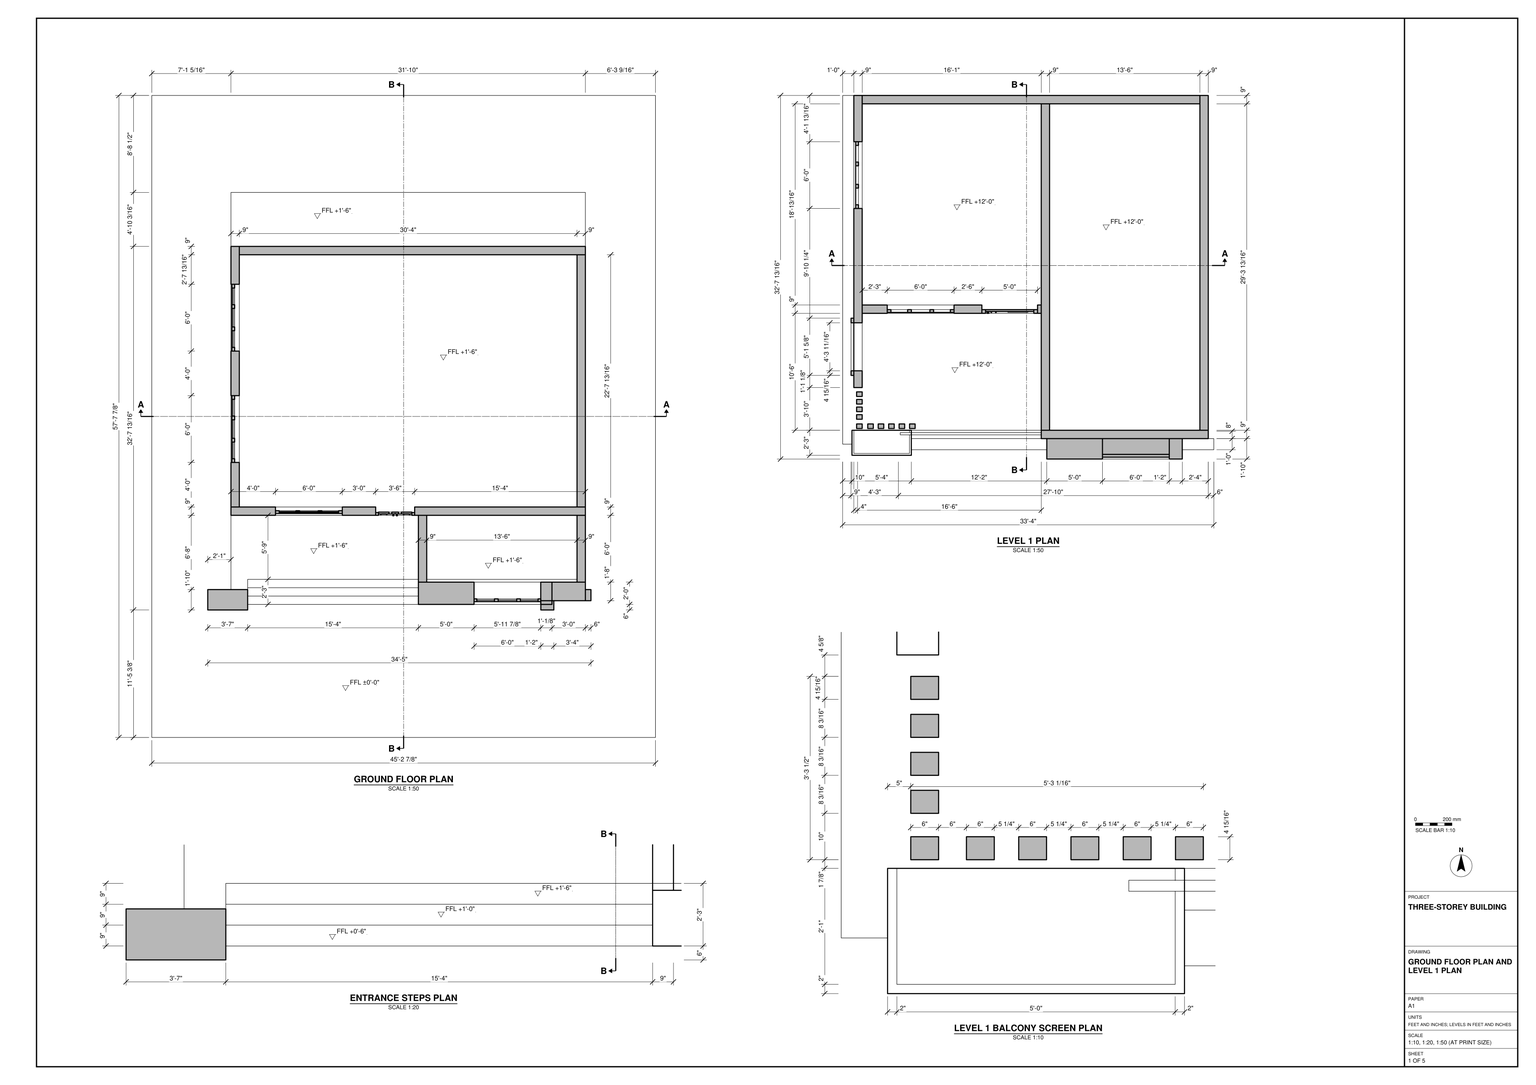
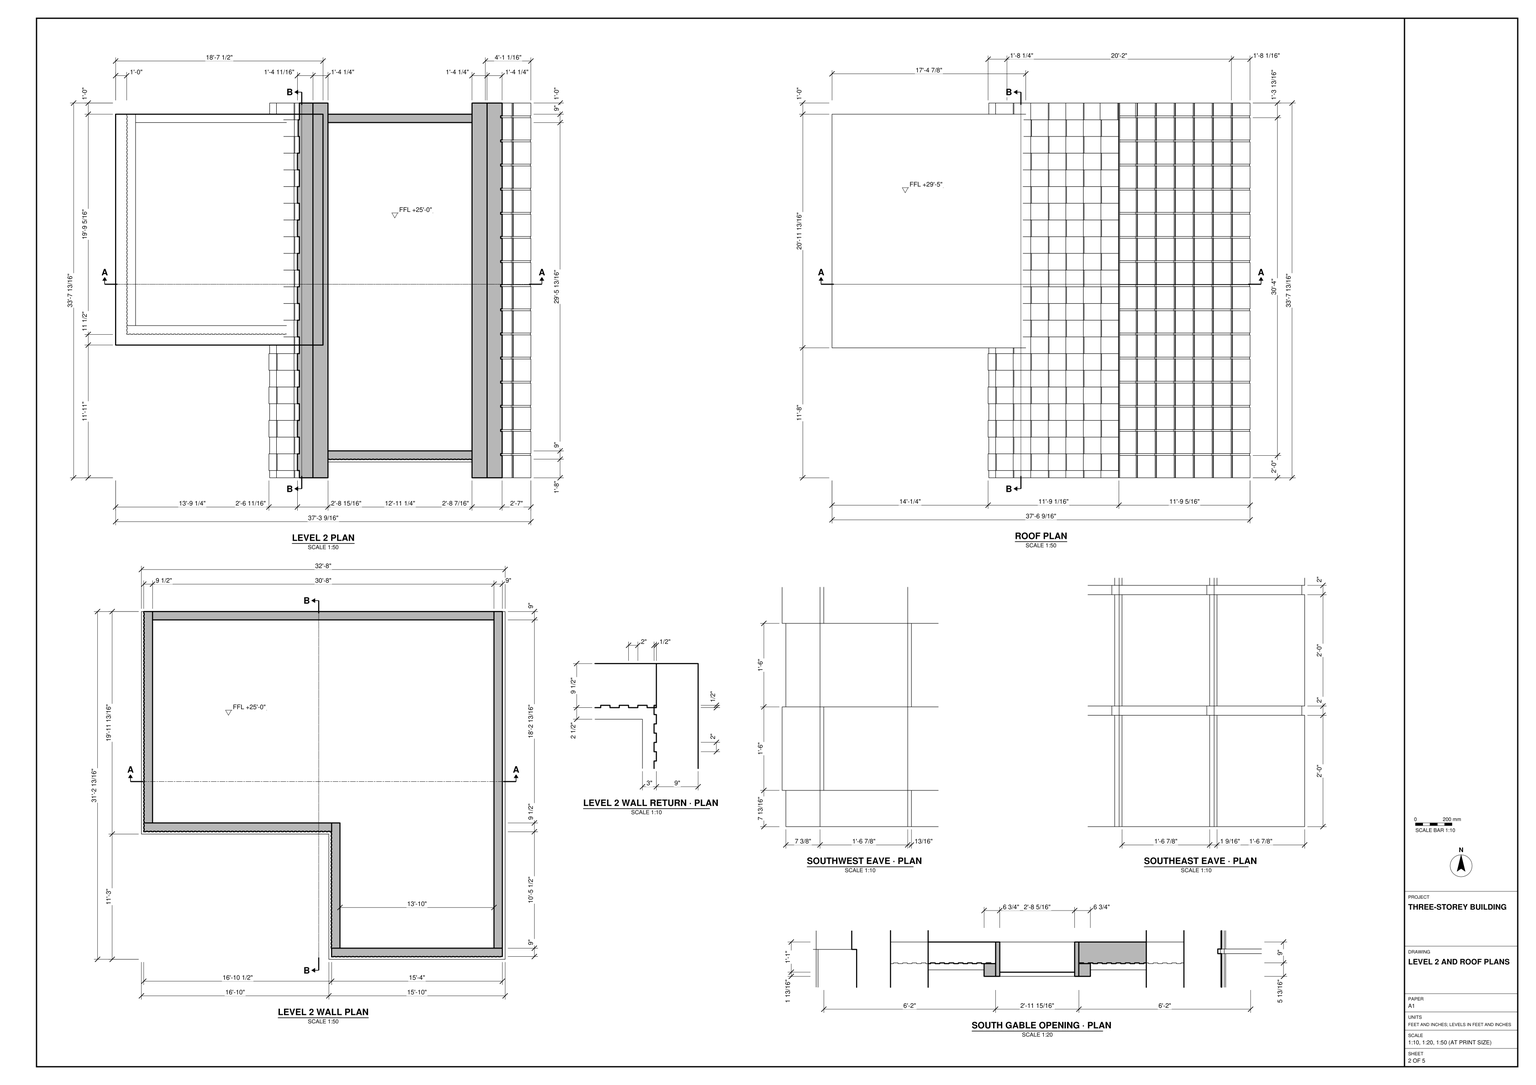
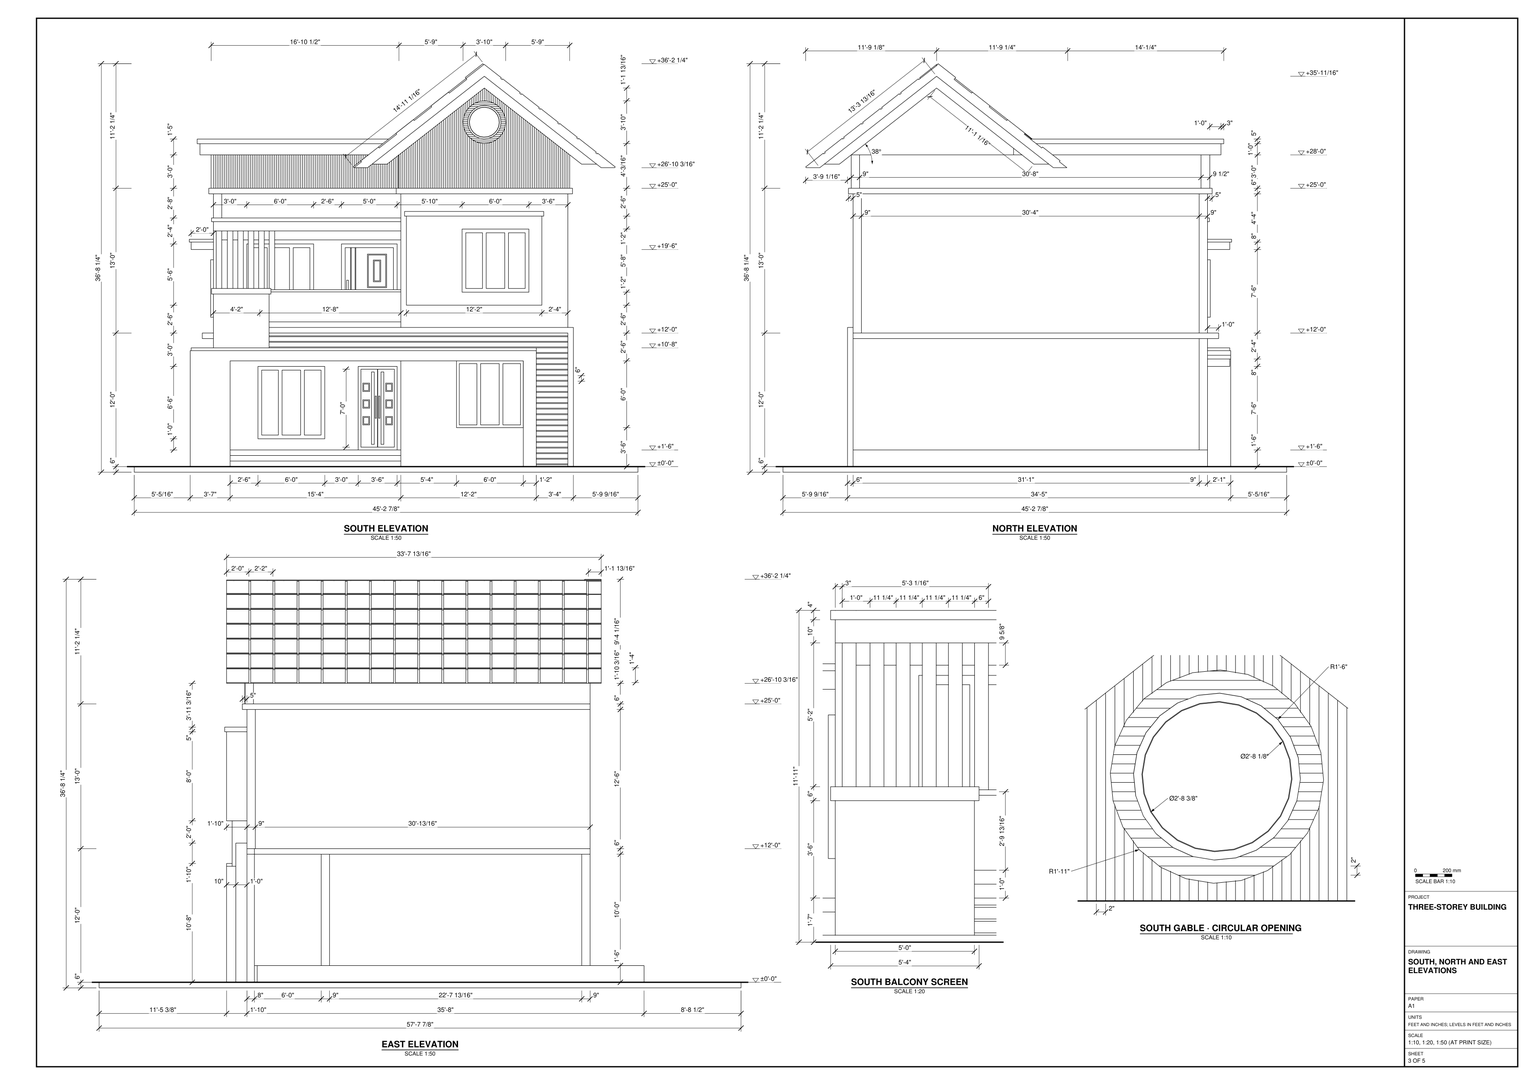
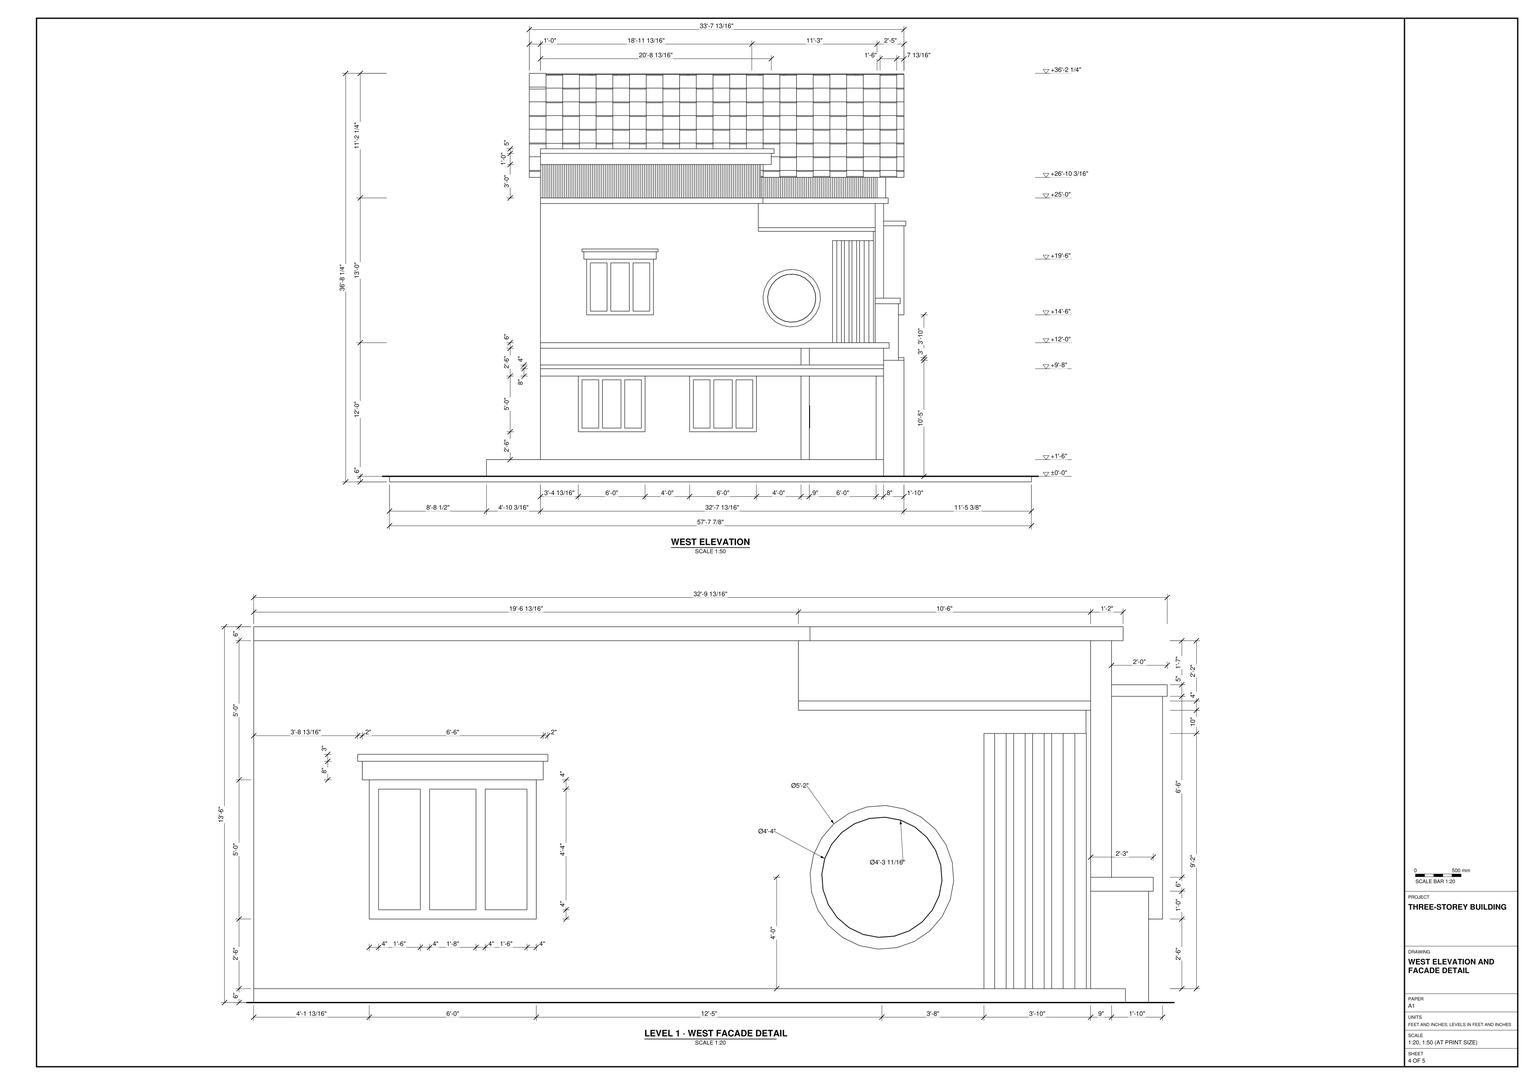
Build the three-storey building and its rectangular site base in SketchUp using task_files/diagram_01.pdf. Work in feet and inches. Including the base, the model is 45'-2 7/8" wide, 57'-7 7/8" deep and 36'-8 1/4" high. Use ±0'-0" as the ground datum, with Level 1 at +12'-0" and Level 2 at +25'-0". The entrance steps rise from the ground datum to the raised ground floor at +1'-6".

Set out the floor slabs and walls from the plans, keeping the 9" wall thicknesses where marked. On the south side, recess the entrance beside the projecting room and place the doors and windows in their drawn wall planes. At Level 1, model the front balcony with its solid corner base and returning vertical screen. Distinguish the recessed balcony openings from the window in the projecting frame to their right.

Follow the L-shaped Level 2 wall plan. Model the flat roof to the west and the adjoining pitched roof with its ridge running north–south. Include the eave projections, roof divisions and framed circular opening beneath the south gable peak. Keep walls, slabs, roof and any furniture or joinery pieces in separate groups or components, and use components for repeated parts. Any decor or loose items shown may be suitable library components. Save one SketchUp model as output_files/gabled_three_storey_building_with_screened_balcony.skp.

# SketchUp Ruby script. Lengths in inches.
U = 1.inch
M = Sketchup.active_model
def pt(a) = Geom::Point3d.new(a.map { |v| v * U })
def face(e, loops, mat)
  f = e.add_face(loops[0].map { |a| pt(a) })
  loops[1..].each { |l| e.add_face(l.map { |a| pt(a) }).erase! }
  f.material = f.back_material = mat if mat
  f
end
# faces: each face lists its corners as indices into pts; further lists are holes
def faces(e, pts, list, mat = nil) = list.each { |f| face(e, (f[0].is_a?(Array) ? f : [f]).map { |l| l.map { |i| pts[i] } }, mat) }
# xy, xz, yz: faces in a plane at the given z, y or x. An outline is a flat list of corners, or four numbers for a rectangle; further outlines are holes
def ring(l) = l.size == 4 ? [[l[0], l[1]], [l[2], l[1]], [l[2], l[3]], [l[0], l[3]]] : l.each_slice(2).to_a
def flat(e, list, mat, &to3) = list.each { |f| face(e, (f[0].is_a?(Array) ? f : [f]).map { |l| ring(l).map { |u, v| to3.(u, v) } }, mat) }
def xy(e, z, list, mat = nil) = flat(e, list, mat) { |x, y| [x, y, z] }
def xz(e, y, list, mat = nil) = flat(e, list, mat) { |x, z| [x, y, z] }
def yz(e, x, list, mat = nil) = flat(e, list, mat) { |y, z| [x, y, z] }
def lines(e, pts, list) = list.each { |a, b| e.add_line(pt(pts[a]), pt(pts[b])) }
# prism: a flat outline (further loops are holes) pulled along v
def prism(e, loops, v, mat = nil)
  f = face(e, loops, mat); d = Geom::Vector3d.new(v.map { |x| x * U })
  f.pushpull(f.normal.samedirection?(d) ? d.length : -d.length)
end
def box(e, o, s, mat = nil) = prism(e, [[o, [o[0] + s[0], o[1], o[2]], [o[0] + s[0], o[1] + s[1], o[2]], [o[0], o[1] + s[1], o[2]]]], [0, 0, s[2]], mat)
def at(x, y, z, deg = 0) = Geom::Transformation.translation(pt([x, y, z])) * Geom::Transformation.rotation(ORIGIN, Z_AXIS, deg.degrees)
def axes(o, x, y, z) = Geom::Transformation.new([*x, 0, *y, 0, *z, 0, *pt(o).to_a, 1])
def part(name) = M.definitions.add(name)
# library, detail: a bought-in or finely detailed component or shape, given as its bounding box
def library(name, o, s) = part(name).tap { |d| box(d.entities, o, s) }
def detail(e, o, s) = box(e.add_group.entities, o, s)
def put(e, d, t, mat = nil) = e.add_instance(d, t).tap { |i| i.material = mat if mat }
def group(e, t, mat = nil) = e.add_group.tap { |g| g.transformation = t; g.material = mat if mat }.entities
root = M.entities
M.materials.add("[Color M00]").color = [255, 255, 255]
M.materials.add("[Color M01]").color = [226, 226, 226]
M.materials.add("[Color M02]").color = [198, 198, 198]
M.materials.add("[Color M03]").color = [170, 170, 170]
M.materials.add("[Color M04]").color = [142, 142, 142]
M.materials.add("[Color M05]").color = [114, 114, 114]
M.materials.add("[Color M06]").color = [86, 86, 86]
M.materials.add("[Metal Silver]").color = [234, 233, 238]
M.materials.add("[Translucent Glass Gray]").color = [128, 128, 128]
M.materials.add("[Wood Cherry Original]").color = [152, 86, 42]
c1 = library("Group\#7",[-5,0,0],[69,0.75,0.75])
c2 = library("Group\#92",[-5,0,0],[69,0.75,0.75])
c3 = library("Group\#93",[-5,0,0],[69,0.75,0.75])
c4 = library("Group\#94",[-5,0,0],[69,0.75,0.75])
c5 = library("Group\#95",[-5,0,0],[69,0.75,0.75])
c6 = library("Group\#96",[-5,0,0],[69,0.75,0.75])
c7 = library("Group\#97",[-5,0,0],[69,0.75,0.75])
c8 = library("Group\#98",[-5,0,0],[69,0.75,0.75])
c9 = library("Group\#99",[-5,0,0],[69,0.75,0.75])
c10 = library("Group\#100",[-5,0,0],[69,0.75,0.75])
c11 = library("Group\#101",[-5,0,0],[69,0.75,0.75])
c12 = library("Group\#13",[0,-0.5,0],[36,2.5,84])
c13 = part("Group\#16")
prism(c13.entities,[[[0,2,23.9375],[0,2,22.2],[0,0.74,22.2],[0,0.74,1.74],[0,2,1.74],[0,2,0],[0,0,0],[0,0,23.9375]]],[1.1875,0,0])
c14 = library("Group\#18",[0,0,0],[64,1.125,1.125])
c15 = library("Group\#25",[0,0,0],[1.125,64,1.125])
c16 = library("Group\#30",[0,0,0],[1,64,1])
c17 = library("Group\#56",[0,0,0],[158,2.375,2.375])
c18 = library("Group\#66",[0,-1,0],[52,3,88])
c19 = part("Group\#73")
box(c19.entities,[0,0,0],[6,4.96,110])
c20 = library("Group\#80",[0,-5.8,-36],[184,14.8,108])
c21 = library("Group\#78",[0,-0.5,0],[45.98,5.5,45.98])
c22 = library("Group\#83",[-0.5,0,0],[9.5,135,36])
c23 = library("Group\#90",[-0.8,0,0],[282.36,403.8125,112.04])
g1 = group(root,at(0,0,0))
box(g1,[0,0,0],[542.875,691.875,6])
g2 = group(root,at(47.33,167.375,6),"[Color M05]")
xy(g2,0,[[38,-8,38,420,420,420,420,3,56,3,56,-8]])
xy(g2,18,[[38,-8,56,-8,56,3,420,3,420,420,38,420]],"[Color M00]")
xz(g2,-8,[[38,0,56,18]])
xz(g2,3,[[56,0,420,18]])
xz(g2,420,[[38,0,420,18]])
yz(g2,38,[[-8,0,420,18]])
yz(g2,56,[[-8,0,3,18]])
yz(g2,420,[[3,0,420,18]])
g3 = group(root,at(47.33,239.375,24),"[Color M01]")
prism(g3,[[[194,9,0],[38,9,0],[38,9,120],[420,9,120],[420,9,0],[236,9,0],[236,9,90],[194,9,90]],[[158,9,90],[86,9,90],[86,9,12],[158,9,12]]],[0,-9,0])
g4 = group(root,at(287.33,143.375,6),"[Color M01]")
xy(g4,0,[[0,0,144,24]])
xy(g4,42,[[60,0,131.9,24]])
xy(g4,114,[[0,0,60,12],[131.9,0,144,12]])
xy(g4,138,[[0,12,60,24],[131.9,12,144,24]])
xz(g4,0,[[0,0,144,0,144,114,131.9,114,131.9,42,60,42,60,114,0,114]])
xz(g4,12,[[0,114,60,138],[131.9,114,144,138]])
xz(g4,24,[[0,0,0,138,60,138,60,42,131.9,42,131.9,138,144,138,144,0]])
yz(g4,0,[[0,0,0,114,12,114,12,138,24,138,24,0]])
yz(g4,60,[[0,42,24,42,24,138,12,138,12,114,0,114]])
yz(g4,131.9,[[0,42,0,114,12,114,12,138,24,138,24,42]])
yz(g4,144,[[0,0,24,0,24,138,12,138,12,114,0,114]])
g5 = group(root,at(287.33,167.375,24))
box(g5,[0,0,0],[9,72,120])
g6 = group(root,at(347.33,146.375,48),"[Wood Cherry Original]")
prism(g6,[[[72,3,0],[0,3,0],[0,3,72],[72,3,72]],[[46,3,3],[46,3,69],[26,3,69],[26,3,3]],[[22,3,3],[22,3,69],[3,3,69],[3,3,3]],[[69,3,69],[50,3,69],[50,3,3],[69,3,3]]],[0,-3,0])
put(root,c1,at(352.33,147.5,114.5))
put(root,c2,at(352.33,147.5,108.5))
put(root,c3,at(352.33,147.5,102.5))
put(root,c4,at(352.33,147.5,96.5))
put(root,c5,at(352.33,147.5,90.5))
put(root,c6,at(352.33,147.5,84.5))
put(root,c7,at(352.33,147.5,78.5))
put(root,c8,at(352.33,147.5,72.5))
put(root,c9,at(352.33,147.5,66.5))
put(root,c10,at(352.33,147.5,60.5))
put(root,c11,at(352.33,147.5,54.5))
g7 = group(root,at(397.33,146.375,51),"[Translucent Glass Gray]")
xz(g7,0,[[0,0,19,66]])
g8 = group(root,at(373.33,146.375,51),"[Translucent Glass Gray]")
xz(g8,0,[[0,0,20,66]])
g9 = group(root,at(350.33,146.375,51),"[Translucent Glass Gray]")
xz(g9,0,[[0,0,19,66]])
g10 = group(root,at(287.33,147.375,6),"[Color M04]")
xy(g10,0,[[144,0,180,20]])
xy(g10,2,[[144,0,180,0.5]])
xy(g10,3,[[144,0,180,0.5]])
xy(g10,8,[[144,0,180,0.5]])
xy(g10,9,[[144,0,180,0.5]])
xy(g10,14,[[144,0,180,0.5]])
xy(g10,15,[[144,0,180,0.5]])
xy(g10,20,[[144,0,180,0.5]])
xy(g10,21,[[144,0,180,0.5]])
xy(g10,26,[[144,0,180,0.5]])
xy(g10,27,[[144,0,180,0.5]])
xy(g10,32,[[144,0,180,0.5]])
xy(g10,33,[[144,0,180,0.5]])
xy(g10,38,[[144,0,180,0.5]])
xy(g10,39,[[144,0,180,0.5]])
xy(g10,44,[[144,0,180,0.5]])
xy(g10,45,[[144,0,180,0.5]])
xy(g10,50,[[144,0,180,0.5]])
xy(g10,51,[[144,0,180,0.5]])
xy(g10,56,[[144,0,180,0.5]])
xy(g10,57,[[144,0,180,0.5]])
xy(g10,62,[[144,0,180,0.5]])
xy(g10,63,[[144,0,180,0.5]])
xy(g10,68,[[144,0,180,0.5]])
xy(g10,69,[[144,0,180,0.5]])
xy(g10,74,[[144,0,180,0.5]])
xy(g10,75,[[144,0,180,0.5]])
xy(g10,80,[[144,0,180,0.5]])
xy(g10,81,[[144,0,180,0.5]])
xy(g10,86,[[144,0,180,0.5]])
xy(g10,87,[[144,0,180,0.5]])
xy(g10,92,[[144,0,180,0.5]])
xy(g10,93,[[144,0,180,0.5]])
xy(g10,98,[[144,0,180,0.5]])
xy(g10,99,[[144,0,180,0.5]])
xy(g10,104,[[144,0,180,0.5]])
xy(g10,105,[[144,0,180,0.5]])
xy(g10,110,[[144,0,180,0.5]])
xy(g10,111,[[144,0,180,0.5]])
xy(g10,114,[[0,0,0,12,60,12,60,20,144,20,144,0]])
xy(g10,116,[[0,0,180,0.5]])
xy(g10,117,[[0,0,180,0.5]])
xy(g10,122,[[0,0,180,0.5]])
xy(g10,123,[[0,0,180,0.5]])
xy(g10,125,[[-154,0,0,12]])
xy(g10,128,[[-154,0,180,0.5]])
xy(g10,129,[[-154,0,180,0.5]])
xy(g10,134,[[-154,0,180,0.5]])
xy(g10,135,[[-154,0,180,0.5]])
xy(g10,140,[[-154,0,180,0.5]])
xy(g10,141,[[-154,0,180,0.5]])
xy(g10,144,[[-154,0,180,0,180,20,60,20,60,12,-154,12]])
xz(g10,0,[[144,0,180,2],[144,3,180,8],[144,9,180,14],[144,15,180,20],[144,21,180,26],
  [144,27,180,32],[144,33,180,38],[144,39,180,44],[144,45,180,50],[144,51,180,56],
  [144,57,180,62],[144,63,180,68],[144,69,180,74],[144,75,180,80],[144,81,180,86],
  [144,87,180,92],[144,93,180,98],[144,99,180,104],[144,105,180,110],[144,111,180,111,180,116,0,116,0,114,144,114],
  [0,117,180,122],[0,123,180,123,180,128,-154,128,-154,125,0,125],[-154,129,180,134],[-154,135,180,140],[-154,141,180,144]])
xz(g10,0.5,[[144,2,180,3],[144,8,180,9],[144,14,180,15],[144,20,180,21],[144,26,180,27],
  [144,32,180,33],[144,38,180,39],[144,44,180,45],[144,50,180,51],[144,56,180,57],
  [144,62,180,63],[144,68,180,69],[144,74,180,75],[144,80,180,81],[144,86,180,87],
  [144,92,180,93],[144,98,180,99],[144,104,180,105],[144,110,180,111],[0,116,180,117],
  [0,122,180,123],[-154,128,180,129],[-154,134,180,135],[-154,140,180,141]])
xz(g10,12,[[0,114,0,125,-154,125,-154,144,60,144,60,114]])
xz(g10,20,[[144,0,144,114,60,114,60,144,180,144,180,0]])
yz(g10,-154,[[0,125,0,128,0.5,128,0.5,129,0,129,0,134,0.5,134,0.5,135,0,135,0,140,0.5,140,0.5,141,0,141,0,144,12,144,12,125]])
yz(g10,0,[[0,114,0,116,0.5,116,0.5,117,0,117,0,122,0.5,122,0.5,123,0,123,0,125,12,125,12,114]])
yz(g10,60,[[12,114,20,144]])
yz(g10,144,[[0,0,0,2,0.5,2,0.5,3,0,3,0,8,0.5,8,0.5,9,0,9,0,14,0.5,14,0.5,15,0,15,0,20,0.5,20,0.5,21,0,21,0,26,0.5,26,0.5,27,0,27,0,32,0.5,32,0.5,33,0,33,0,38,0.5,38,0.5,39,0,39,0,44,0.5,44,0.5,45,0,45,0,50,0.5,50,0.5,51,0,51,0,56,0.5,56,0.5,57,0,57,0,62,0.5,62,0.5,63,0,63,0,68,0.5,68,0.5,69,0,69,0,74,0.5,74,0.5,75,0,75,0,80,0.5,80,0.5,81,0,81,0,86,0.5,86,0.5,87,0,87,0,92,0.5,92,0.5,93,0,93,0,98,0.5,98,0.5,99,0,99,0,104,0.5,104,0.5,105,0,105,0,110,0.5,110,0.5,111,0,111,0,114,20,114,20,0]])
yz(g10,180,[[0,0,20,0,20,144,0,144,0,141,0.5,141,0.5,140,0,140,0,135,0.5,135,0.5,134,0,134,0,129,0.5,129,0.5,128,0,128,0,123,0.5,123,0.5,122,0,122,0,117,0.5,117,0.5,116,0,116,0,111,0.5,111,0.5,110,0,110,0,105,0.5,105,0.5,104,0,104,0,99,0.5,99,0.5,98,0,98,0,93,0.5,93,0.5,92,0,92,0,87,0.5,87,0.5,86,0,86,0,81,0.5,81,0.5,80,0,80,0,75,0.5,75,0.5,74,0,74,0,69,0.5,69,0.5,68,0,68,0,63,0.5,63,0.5,62,0,62,0,57,0.5,57,0.5,56,0,56,0,51,0.5,51,0.5,50,0,50,0,45,0.5,45,0.5,44,0,44,0,39,0.5,39,0.5,38,0,38,0,33,0.5,33,0.5,32,0,32,0,27,0.5,27,0.5,26,0,26,0,21,0.5,21,0.5,20,0,20,0,15,0.5,15,0.5,14,0,14,0,9,0.5,9,0.5,8,0,8,0,3,0.5,3,0.5,2,0,2]])
g11 = group(root,at(241.33,239.375,24),"[Wood Cherry Original]")
prism(g11,[[[42,0,90],[0,0,90],[0,0,0],[42,0,0]],[[3,0,3],[3,0,87],[39,0,87],[39,0,3]]],[0,3,0])
put(root,c12,at(244.33,240.875,27),"[Wood Cherry Original]")
g12 = group(root,at(265.98,240.875,30),"[Translucent Glass Gray]")
xz(g12,0,[[0,0,3,78]])
g13 = group(root,at(255.68,240.875,30),"[Translucent Glass Gray]")
xz(g13,0,[[0,0,3,78]])
put(root,c13,at(259.73,238.875,58.14),"[Metal Silver]")
put(root,c13,at(263.54,238.875,58.14),"[Metal Silver]")
g14 = group(root,at(133.33,241.375,36),"[Wood Cherry Original]")
prism(g14,[[[72,0,78],[0,0,78],[0,0,0],[72,0,0]],[[46,0,4],[26,0,4],[26,0,74],[46,0,74]],[[22,0,74],[22,0,4],[4,0,4],[4,0,74]],[[50,0,4],[50,0,74],[68,0,74],[68,0,4]]],[0,3,0])
put(root,c14,at(137.33,242.3125,107.07))
put(root,c14,at(137.33,242.3125,101.07))
put(root,c14,at(137.33,242.3125,95.07))
put(root,c14,at(137.33,242.3125,89.07))
put(root,c14,at(137.33,242.3125,83.07))
put(root,c14,at(137.33,242.3125,77.07))
put(root,c14,at(137.33,242.3125,71.07))
put(root,c14,at(137.33,242.3125,65.07))
put(root,c14,at(137.33,242.3125,59.07))
put(root,c14,at(137.33,242.3125,53.07))
put(root,c14,at(137.33,242.3125,47.07))
put(root,c14,at(137.33,242.3125,41.07))
put(root,c14,at(137.33,242.3125,35.07))
put(root,c14,at(137.33,242.3125,29.07))
put(root,c14,at(137.33,242.3125,23.07))
put(root,c14,at(137.33,242.3125,17.07))
g15 = group(root,at(183.33,241.375,40),"[Translucent Glass Gray]")
xz(g15,0,[[0,0,18,70]])
g16 = group(root,at(159.33,241.375,40),"[Translucent Glass Gray]")
xz(g16,0,[[0,0,20,70]])
g17 = group(root,at(137.33,241.375,40),"[Translucent Glass Gray]")
xz(g17,0,[[0,0,18,70]])
g18 = group(root,at(85.33,137.375,6),"[Color M05]")
xy(g18,0,[[-25,0,18,22],[334,0,348,10]])
xy(g18,114,[[18,0,18,22,202,22,202,10,334,10,334,0]])
xy(g18,125,[[-25,0,348,0,348,10,202,10,202,22,-25,22]])
xz(g18,0,[[-25,0,18,0,18,114,334,114,334,0,348,0,348,125,-25,125]])
xz(g18,10,[[334,0,334,114,202,114,202,125,348,125,348,0]])
xz(g18,22,[[-25,0,-25,125,202,125,202,114,18,114,18,0]])
yz(g18,-25,[[0,0,22,125]])
yz(g18,18,[[0,0,22,114]])
yz(g18,202,[[10,114,22,125]])
yz(g18,334,[[0,0,10,114]])
yz(g18,348,[[0,0,10,125]])
g19 = group(root,at(85.33,248.375,24),"[Color M01]")
prism(g19,[[[0,280.8125,0],[0,0,0],[0,0,120],[0,280.8125,120]],[[0,48,30],[0,120,30],[0,120,90],[0,48,90]],[[0,240,30],[0,240,90],[0,168,90],[0,168,30]]],[9,0,0])
g20 = group(root,at(86.33,296.375,54),"[Wood Cherry Original]")
prism(g20,[[[0,72,0],[0,0,0],[0,0,60],[0,72,60]],[[0,26,4],[0,46,4],[0,46,56],[0,26,56]],[[0,22,4],[0,22,56],[0,4,56],[0,4,4]],[[0,50,56],[0,50,4],[0,68,4],[0,68,56]]],[3,0,0])
put(root,c15,at(87.27,300.375,104.45))
put(root,c15,at(87.27,300.375,98.45))
put(root,c15,at(87.27,300.375,92.45))
put(root,c15,at(87.27,300.375,86.45))
put(root,c15,at(87.27,300.375,80.45))
put(root,c15,at(87.27,300.375,74.45))
put(root,c15,at(87.27,300.375,68.45))
put(root,c15,at(87.27,300.375,62.45))
put(root,c15,at(87.27,300.375,56.45))
g21 = group(root,at(86.33,300.375,58),"[Translucent Glass Gray]")
yz(g21,0,[[0,0,18,52]])
g22 = group(root,at(86.33,322.375,58),"[Translucent Glass Gray]")
yz(g22,0,[[0,0,20,52]])
g23 = group(root,at(86.33,346.375,58),"[Translucent Glass Gray]")
yz(g23,0,[[0,0,18,52]])
g24 = group(root,at(86.33,416.375,54),"[Wood Cherry Original]")
prism(g24,[[[0,0,60],[0,72,60],[0,72,0],[0,0,0]],[[0,26,56],[0,26,4],[0,46,4],[0,46,56]],[[0,68,56],[0,50,56],[0,50,4],[0,68,4]],[[0,4,4],[0,22,4],[0,22,56],[0,4,56]]],[3,0,0])
put(root,c16,at(87.33,420.375,104.78))
put(root,c16,at(87.33,420.375,98.78))
put(root,c16,at(87.33,420.375,92.78))
put(root,c16,at(87.33,420.375,86.78))
put(root,c16,at(87.33,420.375,80.78))
put(root,c16,at(87.33,420.375,74.78))
put(root,c16,at(87.33,420.375,68.78))
put(root,c16,at(87.33,420.375,62.78))
g25 = group(root,at(86.33,420.375,58),"[Translucent Glass Gray]")
yz(g25,0,[[0,0,18,52]])
g26 = group(root,at(86.33,442.375,58),"[Translucent Glass Gray]")
yz(g26,0,[[0,0,20,52]])
g27 = group(root,at(86.33,466.375,58),"[Translucent Glass Gray]")
yz(g27,0,[[0,0,18,52]])
g28 = group(root,at(94.33,520.1875,24),"[Color M01]")
box(g28,[0,0,0],[373,9,120])
g29 = group(root,at(458.33,248.375,24),"[Color M01]")
box(g29,[0,0,0],[9,271.8125,120])
g30 = group(root,at(61.33,137.375,131),"[Color M05]")
box(g30,[0,0,0],[372,6,3])
g31 = group(root,at(85.33,239.375,144),"[Color M05]")
xy(g31,0,[[-12,-86,-12,289.8125,382,289.8125,382,-80,0,-80,0,-86]])
xy(g31,6,[[-12,-86,0,-86,0,-80,382,-80,382,289.8125,-12,289.8125]],"[Color M00]")
xz(g31,-86,[[-12,0,0,6]])
xz(g31,-80,[[0,0,382,6]])
xz(g31,289.8125,[[-12,0,382,6]])
yz(g31,-12,[[-86,0,289.8125,6]])
yz(g31,0,[[-86,0,-80,6]])
yz(g31,382,[[-80,0,289.8125,6]])
g32 = group(root,at(208.08,147.375,6))
prism(g32,[[[-74.75,0,144],[259.25,0,144],[259.25,0,0],[265.25,0,0],[265.25,0,150],[-74.75,0,150]]],[0,12,0])
g33 = group(root,at(61.33,167.375,126))
box(g33,[24,-8,0],[202,80,18])
g34 = group(root,at(61.33,239.375,114))
box(g34,[0,-80,0],[24,369.8125,8])
g35 = group(root,at(60.33,239.375,122),"[Color M05]")
box(g35,[0,-80,0],[25,369.8125,4])
g36 = group(root,at(85.33,143.375,131),"[Color M02]")
xy(g36,0,[[0,0,60,16]])
xy(g36,19,[[0,16,4,25]])
xy(g36,31,[[4,16,60,25]])
xy(g36,61,[[0,0,60,25]])
xz(g36,0,[[0,0,60,61]])
xz(g36,16,[[0,0,0,19,4,19,4,31,60,31,60,0]])
xz(g36,25,[[0,19,0,61,60,61,60,31,4,31,4,19]])
yz(g36,0,[[0,0,0,61,25,61,25,19,16,19,16,0]])
yz(g36,4,[[16,19,25,31]])
yz(g36,60,[[0,0,16,0,16,31,25,31,25,61,0,61]])
g37 = group(root,at(458.33,167.375,24),"[Color M01]")
box(g37,[0,0,0],[9,72,120])
g38 = group(root,at(287.33,159.375,150),"[Color M01]")
box(g38,[0,0,0],[180,9,150])
g39 = group(root,at(287.33,168.375,150),"[Color M01]")
box(g39,[0,0,0],[9,351.8125,150])
g40 = group(root,at(458.33,168.375,150),"[Color M01]")
box(g40,[0,0,0],[9,360.8125,150])
g41 = group(root,at(76.33,294.375,150),"[Color M01]")
prism(g41,[[[211,9,0],[207,9,0],[207,9,96],[147,9,96],[147,9,0],[18,9,0],[18,9,150],[211,9,150]],[[117,9,96],[45,9,96],[45,9,30],[117,9,30]]],[0,-9,0])
g42 = group(root,at(85.33,255.375,150),"[Color M01]")
xy(g42,0,[[0,-41,9,273.8125]])
xy(g42,30,[[0,152,9,224]])
xy(g42,90,[[0,152,9,224]])
xy(g42,110,[[0,-85,0,-41,9,-41,9,39,202,39,202,-85]])
xy(g42,120,[[0,-85,202,39]])
xy(g42,150,[[0,39,9,273.8125]])
xz(g42,-85,[[0,110,202,120]])
xz(g42,-41,[[0,0,9,110]])
xz(g42,39,[[9,110,202,120],[0,120,9,150]])
xz(g42,152,[[0,30,9,90]])
xz(g42,224,[[0,30,9,90]])
xz(g42,273.8125,[[0,0,9,150]])
yz(g42,-3,[[[4.67,17.04,-3.4,17.67,-11.03,20.36,-17.71,24.93,-22.97,31.08,-26.47,38.38,-27.96,46.33,-27.33,54.4,-24.64,62.03,-20.07,68.71,-13.92,73.97,-6.62,77.47,1.33,78.96,9.4,78.33,17.03,75.64,23.71,71.07,28.97,64.92,32.47,57.62,33.96,49.67,33.33,41.6,30.64,33.97,26.07,27.29,19.92,22.03,12.62,18.53],[4.4,22.04,11.07,23.28,17.19,26.22,22.35,30.63,26.18,36.23,28.44,42.63,28.96,49.4,27.72,56.07,24.78,62.19,20.37,67.35,14.77,71.18,8.37,73.44,1.6,73.96,-5.07,72.72,-11.19,69.78,-16.35,65.37,-20.18,59.77,-22.44,53.37,-22.96,46.6,-21.72,39.93,-18.78,33.81,-14.37,28.65,-8.77,24.82,-2.37,22.56]]],"[Color M04]")
yz(g42,0,[[[-41,0,-41,110,-85,110,-85,120,39,120,39,150,273.8125,150,273.8125,0],[152,30,224,90],[4.67,17.04,12.62,18.53,19.92,22.03,26.07,27.29,30.64,33.97,33.33,41.6,33.96,49.67,32.47,57.62,28.97,64.92,23.71,71.07,17.03,75.64,9.4,78.33,1.33,78.96,-6.62,77.47,-13.92,73.97,-20.07,68.71,-24.64,62.03,-27.33,54.4,-27.96,46.33,-26.47,38.38,-22.97,31.08,-17.71,24.93,-11.03,20.36,-3.4,17.67]],[[4.67,17.04,-3.4,17.67,-11.03,20.36,-17.71,24.93,-22.97,31.08,-26.47,38.38,-27.96,46.33,-27.33,54.4,-24.64,62.03,-20.07,68.71,-13.92,73.97,-6.62,77.47,1.33,78.96,9.4,78.33,17.03,75.64,23.71,71.07,28.97,64.92,32.47,57.62,33.96,49.67,33.33,41.6,30.64,33.97,26.07,27.29,19.92,22.03,12.62,18.53],[4.4,22.04,11.07,23.28,17.19,26.22,22.35,30.63,26.18,36.23,28.44,42.63,28.96,49.4,27.72,56.07,24.78,62.19,20.37,67.35,14.77,71.18,8.37,73.44,1.6,73.96,-5.07,72.72,-11.19,69.78,-16.35,65.37,-20.18,59.77,-22.44,53.37,-22.96,46.6,-21.72,39.93,-18.78,33.81,-14.37,28.65,-8.77,24.82,-2.37,22.56]]])
yz(g42,0,[[4.39,22.18,11.03,23.42,17.12,26.33,22.24,30.73,26.06,36.29,28.3,42.66,28.82,49.39,27.58,56.03,24.67,62.12,20.27,67.24,14.71,71.06,8.34,73.3,1.61,73.82,-5.03,72.58,-11.12,69.67,-16.24,65.27,-20.06,59.71,-22.3,53.34,-22.82,46.61,-21.58,39.97,-18.67,33.88,-14.27,28.76,-8.71,24.94,-2.34,22.7]],"[Translucent Glass Gray]")
yz(g42,9,[[[-41,0,273.8125,0,273.8125,150,39,150,39,110,-41,110],[152,30,224,90],[4.4,22.04,-2.37,22.56,-8.77,24.82,-14.37,28.65,-18.78,33.81,-21.72,39.93,-22.96,46.6,-22.44,53.37,-20.18,59.77,-16.35,65.37,-11.19,69.78,-5.07,72.72,1.6,73.96,8.37,73.44,14.77,71.18,20.37,67.35,24.78,62.19,27.72,56.07,28.96,49.4,28.44,42.63,26.18,36.23,22.35,30.63,17.19,26.22,11.07,23.28]]])
yz(g42,202,[[-85,110,39,120]])
p = [[0,4.67,17.04],[0,-3.4,17.67],[-3,-3.4,17.67],[-3,4.67,17.04],[0,12.62,18.53],[-3,12.62,18.53],
  [0,-11.03,20.36],[-3,-11.03,20.36],[0,19.92,22.03],[-3,19.92,22.03],[0,-17.71,24.93],[-3,-17.71,24.93],
  [0,-2.37,22.56],[0,4.4,22.04],[-3,4.4,22.04],[-3,-2.37,22.56],[9,-2.37,22.56],[9,4.4,22.04],
  [0,11.07,23.28],[-3,11.07,23.28],[9,11.07,23.28],[0,26.07,27.29],[-3,26.07,27.29],[0,-8.77,24.82],
  [-3,-8.77,24.82],[9,-8.77,24.82],[0,17.19,26.22],[-3,17.19,26.22],[9,17.19,26.22],[0,-14.37,28.65],
  [-3,-14.37,28.65],[9,-14.37,28.65],[0,-22.97,31.08],[-3,-22.97,31.08],[0,22.35,30.63],[-3,22.35,30.63],
  [9,22.35,30.63],[0,30.64,33.97],[-3,30.64,33.97],[0,-18.78,33.81],[-3,-18.78,33.81],[9,-18.78,33.81],
  [0,26.18,36.23],[-3,26.18,36.23],[9,26.18,36.23],[0,-26.47,38.38],[-3,-26.47,38.38],[0,-21.72,39.93],
  [-3,-21.72,39.93],[9,-21.72,39.93],[0,33.33,41.6],[-3,33.33,41.6],[0,28.44,42.63],[-3,28.44,42.63],
  [9,28.44,42.63],[0,-27.96,46.33],[-3,-27.96,46.33],[0,-22.96,46.6],[-3,-22.96,46.6],[9,-22.96,46.6],
  [0,33.96,49.67],[-3,33.96,49.67],[0,28.96,49.4],[-3,28.96,49.4],[9,28.96,49.4],[0,-27.33,54.4],
  [-3,-27.33,54.4],[0,-22.44,53.37],[-3,-22.44,53.37],[9,-22.44,53.37],[0,27.72,56.07],[-3,27.72,56.07],
  [9,27.72,56.07],[0,32.47,57.62],[-3,32.47,57.62],[0,-20.18,59.77],[-3,-20.18,59.77],[9,-20.18,59.77],
  [0,-24.64,62.03],[-3,-24.64,62.03],[0,24.78,62.19],[-3,24.78,62.19],[9,24.78,62.19],[0,28.97,64.92],
  [-3,28.97,64.92],[0,-16.35,65.37],[-3,-16.35,65.37],[9,-16.35,65.37],[0,-20.07,68.71],[-3,-20.07,68.71],
  [0,20.37,67.35],[-3,20.37,67.35],[9,20.37,67.35],[0,23.71,71.07],[-3,23.71,71.07],[0,-11.19,69.78],
  [-3,-11.19,69.78],[9,-11.19,69.78],[0,14.77,71.18],[-3,14.77,71.18],[9,14.77,71.18],[0,-13.92,73.97],
  [-3,-13.92,73.97],[0,-5.07,72.72],[-3,-5.07,72.72],[9,-5.07,72.72],[0,17.03,75.64],[-3,17.03,75.64],
  [0,8.37,73.44],[-3,8.37,73.44],[9,8.37,73.44],[0,1.6,73.96],[-3,1.6,73.96],[9,1.6,73.96],
  [0,-6.62,77.47],[-3,-6.62,77.47],[0,9.4,78.33],[-3,9.4,78.33],[0,1.33,78.96],[-3,1.33,78.96]]
faces(g42,p,[[0,1,2,3],[4,0,3,5],[1,6,7,2],[8,4,5,9],[6,10,11,7],[12,13,14,15],[13,18,19,14],[21,8,9,22],
  [23,12,15,24],[18,26,27,19],[29,23,24,30],[10,32,33,11],[26,34,35,27],[37,21,22,38],[39,29,30,40],[34,42,43,35],
  [32,45,46,33],[47,39,40,48],[50,37,38,51],[42,52,53,43],[45,55,56,46],[57,47,48,58],[60,50,51,61],[52,62,63,53],
  [55,65,66,56],[67,57,58,68],[62,70,71,63],[73,60,61,74],[75,67,68,76],[65,78,79,66],[70,80,81,71],[83,73,74,84],
  [85,75,76,86],[78,88,89,79],[80,90,91,81],[93,83,84,94],[95,85,86,96],[90,98,99,91],[88,101,102,89],[103,95,96,104],
  [106,93,94,107],[98,108,109,99],[111,103,104,112],[108,111,112,109],[101,114,115,102],[116,106,107,117],[114,118,119,115],[118,116,117,119]],"[Color M04]")
faces(g42,p,[[13,12,16,17],[18,13,17,20],[12,23,25,16],[26,18,20,28],[23,29,31,25],[34,26,28,36],[29,39,41,31],[42,34,36,44],
  [39,47,49,41],[52,42,44,54],[47,57,59,49],[62,52,54,64],[57,67,69,59],[70,62,64,72],[67,75,77,69],[80,70,72,82],
  [75,85,87,77],[90,80,82,92],[85,95,97,87],[98,90,92,100],[95,103,105,97],[108,98,100,110],[103,111,113,105],[111,108,110,113]])
g43 = group(root,at(85.33,159.375,150),"[Color M05]")
box(g43,[4,0,0],[198,9,12])
g44 = group(root,at(293.33,137.375,180),"[Color M04]")
prism(g44,[[[0,0,96],[0,0,0],[146,0,0],[146,0,96]],[[60,0,14],[60,0,82],[132,0,82],[132,0,14]]],[0,22,0])
g45 = group(root,at(353.33,139.375,194),"[Wood Cherry Original]")
prism(g45,[[[0,3,68],[72,3,68],[72,3,0],[0,3,0]],[[26,3,4],[46,3,4],[46,3,64],[26,3,64]],[[22,3,4],[22,3,64],[4,3,64],[4,3,4]],[[50,3,64],[50,3,4],[68,3,4],[68,3,64]]],[0,-3,0])
g46 = group(root,at(403.33,139.375,198),"[Translucent Glass Gray]")
xz(g46,0,[[0,0,18,60]])
g47 = group(root,at(379.33,139.375,198),"[Translucent Glass Gray]")
xz(g47,0,[[0,0,20,60]])
g48 = group(root,at(357.33,139.375,198),"[Translucent Glass Gray]")
xz(g48,0,[[0,0,18,60]])
g49 = group(root,at(83.33,141.375,192))
box(g49,[0,0,0],[64,27,6])
put(root,c17,at(135.33,163.4375,194.32),"[Metal Silver]")
g50 = group(root,at(135.33,164.625,162),"[Translucent Glass Gray]")
xz(g50,0,[[0,0,152,33.84]])
g51 = group(root,at(85.33,520.1875,150),"[Color M01]")
box(g51,[9,0,0],[364,9,150])
g52 = group(root,at(87.33,407.375,180),"[Wood Cherry Original]")
prism(g52,[[[0,0,60],[0,72,60],[0,72,0],[0,0,0]],[[0,26,4],[0,46,4],[0,46,56],[0,26,56]],[[0,22,4],[0,22,56],[0,4,56],[0,4,4]],[[0,50,56],[0,50,4],[0,68,4],[0,68,56]]],[3,0,0])
g53 = group(root,at(87.33,411.375,184),"[Translucent Glass Gray]")
yz(g53,0,[[0,0,18,52]])
g54 = group(root,at(87.33,433.375,184),"[Translucent Glass Gray]")
yz(g54,0,[[0,0,20,52]])
g55 = group(root,at(87.33,457.375,184),"[Translucent Glass Gray]")
yz(g55,0,[[0,0,18,52]])
g56 = group(root,at(61.33,404.375,240))
box(g56,[0,0,0],[24,78,8])
g57 = group(root,at(59.33,402.375,248),"[Color M05]")
box(g57,[0,0,0],[26,82,3])
g58 = group(root,at(223.33,294.375,150),"[Wood Cherry Original]")
prism(g58,[[[60,4,0],[0,4,0],[0,4,96],[60,4,96]],[[4,4,4],[56,4,4],[56,4,92],[4,4,92]]],[0,-4,0])
put(root,c18,at(227.33,296.375,154),"[Wood Cherry Original]")
g59 = group(root,at(228.84,294.375,180.41),"[Metal Silver]")
prism(g59,[[[2.0625,2,24.7],[2.0625,2,26.4375],[2.0625,0,26.4375],[2.0625,0,0],[2.0625,2,0],[2.0625,2,1.73],[2.0625,0.73,1.73],[2.0625,0.73,24.7]]],[-2.0625,0,0])
g60 = group(root,at(121.33,295.375,180),"[Wood Cherry Original]")
prism(g60,[[[0,3,66],[72,3,66],[72,3,0],[0,3,0]],[[26,3,4],[46,3,4],[46,3,62],[26,3,62]],[[22,3,4],[22,3,62],[4,3,62],[4,3,4]],[[50,3,62],[50,3,4],[68,3,4],[68,3,62]]],[0,-3,0])
g61 = group(root,at(171.33,295.375,184),"[Translucent Glass Gray]")
xz(g61,0,[[0,0,18,58]])
g62 = group(root,at(147.33,295.375,184),"[Translucent Glass Gray]")
xz(g62,0,[[0,0,20,58]])
g63 = group(root,at(125.33,295.375,184),"[Translucent Glass Gray]")
xz(g63,0,[[0,0,18,58]])
put(root,c19,at(88.33,204.8,150),"[Color M05]")
put(root,c19,at(88.33,196.61,150),"[Color M05]")
put(root,c19,at(88.33,188.42,150),"[Color M05]")
put(root,c19,at(88.33,180.24,150),"[Color M05]")
put(root,c19,at(100.33,170.24,150),"[Color M05]")
put(root,c19,at(111.6,170.24,150),"[Color M05]")
put(root,c19,at(122.86,170.24,150),"[Color M05]")
put(root,c19,at(134.13,170.24,150),"[Color M05]")
put(root,c19,at(145.39,170.24,150),"[Color M05]")
g64 = group(root,at(85.33,177.375,270),"[Color M03]")
box(g64,[-2,-9,0],[204,126,4])
put(root,c19,at(88.33,170.24,150),"[Color M05]")
g65 = group(root,at(80.33,154.375,300))
prism(g65,[[[0,135,0],[0,374.8125,0],[392,374.8125,0],[392,0,0],[202,0,0],[202,135,0]]],[0,0,6])
g66 = group(root,at(83.33,301.375,306),"[Color M04]")
prism(g66,[[[9,227.8125,0],[9,0,0],[0,0,0],[0,1.8125,0],[-0.5,1.8125,0],[-0.5,3.8125,0],[0,3.8125,0],[0,5.8125,0],[-0.5,5.8125,0],[-0.5,7.8125,0],[0,7.8125,0],[0,9.8125,0],[-0.5,9.8125,0],[-0.5,11.8125,0],[0,11.8125,0],[0,13.8125,0],[-0.5,13.8125,0],[-0.5,15.8125,0],[0,15.8125,0],[0,17.8125,0],[-0.5,17.8125,0],[-0.5,19.8125,0],[0,19.8125,0],[0,21.8125,0],[-0.5,21.8125,0],[-0.5,23.8125,0],[0,23.8125,0],[0,25.8125,0],[-0.5,25.8125,0],[-0.5,27.8125,0],[0,27.8125,0],[0,29.8125,0],[-0.5,29.8125,0],[-0.5,31.8125,0],[0,31.8125,0],[0,33.8125,0],[-0.5,33.8125,0],[-0.5,35.8125,0],[0,35.8125,0],[0,37.8125,0],[-0.5,37.8125,0],[-0.5,39.8125,0],[0,39.8125,0],[0,41.8125,0],[-0.5,41.8125,0],[-0.5,43.8125,0],[0,43.8125,0],[0,45.8125,0],[-0.5,45.8125,0],[-0.5,47.8125,0],[0,47.8125,0],[0,49.8125,0],[-0.5,49.8125,0],[-0.5,51.8125,0],[0,51.8125,0],[0,53.8125,0],[-0.5,53.8125,0],[-0.5,55.8125,0],[0,55.8125,0],[0,57.8125,0],[-0.5,57.8125,0],[-0.5,59.8125,0],[0,59.8125,0],[0,61.8125,0],[-0.5,61.8125,0],[-0.5,63.8125,0],[0,63.8125,0],[0,65.8125,0],[-0.5,65.8125,0],[-0.5,67.8125,0],[0,67.8125,0],[0,69.8125,0],[-0.5,69.8125,0],[-0.5,71.8125,0],[0,71.8125,0],[0,73.8125,0],[-0.5,73.8125,0],[-0.5,75.8125,0],[0,75.8125,0],[0,77.8125,0],[-0.5,77.8125,0],[-0.5,79.8125,0],[0,79.8125,0],[0,81.8125,0],[-0.5,81.8125,0],[-0.5,83.8125,0],[0,83.8125,0],[0,85.8125,0],[-0.5,85.8125,0],[-0.5,87.8125,0],[0,87.8125,0],[0,89.8125,0],[-0.5,89.8125,0],[-0.5,91.8125,0],[0,91.8125,0],[0,93.8125,0],[-0.5,93.8125,0],[-0.5,95.8125,0],[0,95.8125,0],[0,97.8125,0],[-0.5,97.8125,0],[-0.5,99.8125,0],[0,99.8125,0],[0,101.8125,0],[-0.5,101.8125,0],[-0.5,103.8125,0],[0,103.8125,0],[0,105.8125,0],[-0.5,105.8125,0],[-0.5,107.8125,0],[0,107.8125,0],[0,109.8125,0],[-0.5,109.8125,0],[-0.5,111.8125,0],[0,111.8125,0],[0,113.8125,0],[-0.5,113.8125,0],[-0.5,115.8125,0],[0,115.8125,0],[0,117.8125,0],[-0.5,117.8125,0],[-0.5,119.8125,0],[0,119.8125,0],[0,121.8125,0],[-0.5,121.8125,0],[-0.5,123.8125,0],[0,123.8125,0],[0,125.8125,0],[-0.5,125.8125,0],[-0.5,127.8125,0],[0,127.8125,0],[0,129.8125,0],[-0.5,129.8125,0],[-0.5,131.8125,0],[0,131.8125,0],[0,133.8125,0],[-0.5,133.8125,0],[-0.5,135.8125,0],[0,135.8125,0],[0,137.8125,0],[-0.5,137.8125,0],[-0.5,139.8125,0],[0,139.8125,0],[0,141.8125,0],[-0.5,141.8125,0],[-0.5,143.8125,0],[0,143.8125,0],[0,145.8125,0],[-0.5,145.8125,0],[-0.5,147.8125,0],[0,147.8125,0],[0,149.8125,0],[-0.5,149.8125,0],[-0.5,151.8125,0],[0,151.8125,0],[0,153.8125,0],[-0.5,153.8125,0],[-0.5,155.8125,0],[0,155.8125,0],[0,157.8125,0],[-0.5,157.8125,0],[-0.5,159.8125,0],[0,159.8125,0],[0,161.8125,0],[-0.5,161.8125,0],[-0.5,163.8125,0],[0,163.8125,0],[0,165.8125,0],[-0.5,165.8125,0],[-0.5,167.8125,0],[0,167.8125,0],[0,169.8125,0],[-0.5,169.8125,0],[-0.5,171.8125,0],[0,171.8125,0],[0,173.8125,0],[-0.5,173.8125,0],[-0.5,175.8125,0],[0,175.8125,0],[0,177.8125,0],[-0.5,177.8125,0],[-0.5,179.8125,0],[0,179.8125,0],[0,181.8125,0],[-0.5,181.8125,0],[-0.5,183.8125,0],[0,183.8125,0],[0,185.8125,0],[-0.5,185.8125,0],[-0.5,187.8125,0],[0,187.8125,0],[0,189.8125,0],[-0.5,189.8125,0],[-0.5,191.8125,0],[0,191.8125,0],[0,193.8125,0],[-0.5,193.8125,0],[-0.5,195.8125,0],[0,195.8125,0],[0,197.8125,0],[-0.5,197.8125,0],[-0.5,199.8125,0],[0,199.8125,0],[0,201.8125,0],[-0.5,201.8125,0],[-0.5,203.8125,0],[0,203.8125,0],[0,205.8125,0],[-0.5,205.8125,0],[-0.5,207.8125,0],[0,207.8125,0],[0,209.8125,0],[-0.5,209.8125,0],[-0.5,211.8125,0],[0,211.8125,0],[0,213.8125,0],[-0.5,213.8125,0],[-0.5,215.8125,0],[0,215.8125,0],[0,217.8125,0],[-0.5,217.8125,0],[-0.5,219.8125,0],[0,219.8125,0],[0,221.8125,0],[-0.5,221.8125,0],[-0.5,223.8125,0],[0,223.8125,0],[0,225.8125,0],[-0.5,225.8125,0],[-0.5,227.8125,0]]],[0,0,36])
g67 = group(root,at(83.33,292.375,306),"[Color M04]")
prism(g67,[[[2,-0.5,0],[-0.5,-0.5,0],[-0.5,1,0],[0,1,0],[0,3,0],[-0.5,3,0],[-0.5,5,0],[0,5,0],[0,7,0],[-0.5,7,0],[-0.5,9,0],[202,9,0],[202,-0.5,0],[200,-0.5,0],[200,0,0],[198,0,0],[198,-0.5,0],[196,-0.5,0],[196,0,0],[194,0,0],[194,-0.5,0],[192,-0.5,0],[192,0,0],[190,0,0],[190,-0.5,0],[188,-0.5,0],[188,0,0],[186,0,0],[186,-0.5,0],[184,-0.5,0],[184,0,0],[182,0,0],[182,-0.5,0],[180,-0.5,0],[180,0,0],[178,0,0],[178,-0.5,0],[176,-0.5,0],[176,0,0],[174,0,0],[174,-0.5,0],[172,-0.5,0],[172,0,0],[170,0,0],[170,-0.5,0],[168,-0.5,0],[168,0,0],[166,0,0],[166,-0.5,0],[164,-0.5,0],[164,0,0],[162,0,0],[162,-0.5,0],[160,-0.5,0],[160,0,0],[158,0,0],[158,-0.5,0],[156,-0.5,0],[156,0,0],[154,0,0],[154,-0.5,0],[152,-0.5,0],[152,0,0],[150,0,0],[150,-0.5,0],[148,-0.5,0],[148,0,0],[146,0,0],[146,-0.5,0],[144,-0.5,0],[144,0,0],[142,0,0],[142,-0.5,0],[140,-0.5,0],[140,0,0],[138,0,0],[138,-0.5,0],[136,-0.5,0],[136,0,0],[134,0,0],[134,-0.5,0],[132,-0.5,0],[132,0,0],[130,0,0],[130,-0.5,0],[128,-0.5,0],[128,0,0],[126,0,0],[126,-0.5,0],[124,-0.5,0],[124,0,0],[122,0,0],[122,-0.5,0],[120,-0.5,0],[120,0,0],[118,0,0],[118,-0.5,0],[116,-0.5,0],[116,0,0],[114,0,0],[114,-0.5,0],[112,-0.5,0],[112,0,0],[110,0,0],[110,-0.5,0],[108,-0.5,0],[108,0,0],[106,0,0],[106,-0.5,0],[104,-0.5,0],[104,0,0],[102,0,0],[102,-0.5,0],[100,-0.5,0],[100,0,0],[98,0,0],[98,-0.5,0],[96,-0.5,0],[96,0,0],[94,0,0],[94,-0.5,0],[92,-0.5,0],[92,0,0],[90,0,0],[90,-0.5,0],[88,-0.5,0],[88,0,0],[86,0,0],[86,-0.5,0],[84,-0.5,0],[84,0,0],[82,0,0],[82,-0.5,0],[80,-0.5,0],[80,0,0],[78,0,0],[78,-0.5,0],[76,-0.5,0],[76,0,0],[74,0,0],[74,-0.5,0],[72,-0.5,0],[72,0,0],[70,0,0],[70,-0.5,0],[68,-0.5,0],[68,0,0],[66,0,0],[66,-0.5,0],[64,-0.5,0],[64,0,0],[62,0,0],[62,-0.5,0],[60,-0.5,0],[60,0,0],[58,0,0],[58,-0.5,0],[56,-0.5,0],[56,0,0],[54,0,0],[54,-0.5,0],[52,-0.5,0],[52,0,0],[50,0,0],[50,-0.5,0],[48,-0.5,0],[48,0,0],[46,0,0],[46,-0.5,0],[44,-0.5,0],[44,0,0],[42,0,0],[42,-0.5,0],[40,-0.5,0],[40,0,0],[38,0,0],[38,-0.5,0],[36,-0.5,0],[36,0,0],[34,0,0],[34,-0.5,0],[32,-0.5,0],[32,0,0],[30,0,0],[30,-0.5,0],[28,-0.5,0],[28,0,0],[26,0,0],[26,-0.5,0],[24,-0.5,0],[24,0,0],[22,0,0],[22,-0.5,0],[20,-0.5,0],[20,0,0],[18,0,0],[18,-0.5,0],[16,-0.5,0],[16,0,0],[14,0,0],[14,-0.5,0],[12,-0.5,0],[12,0,0],[10,0,0],[10,-0.5,0],[8,-0.5,0],[8,0,0],[6,0,0],[6,-0.5,0],[4,-0.5,0],[4,0,0],[2,0,0]]],[0,0,36])
g68 = group(root,at(256.33,157.375,332))
prism(g68,[[[225.78,-20,0],[242.01,-20,0],[121,-20,94.7],[0,-20,0],[16.23,-20,0],[29,-20,10],[121,-20,82],[213,-20,10]]],[0,403.8125,0])
put(root,c20,at(285.33,157.375,342),"[Color M04]")
put(root,c21,at(354.34,152.08,354.21),"[Color M05]")
g69 = group(root,at(460.33,166.375,306),"[Color M01]")
box(g69,[0,0,0],[9,362.8125,36])
g70 = group(root,at(92.33,520.1875,306),"[Color M01]")
box(g70,[0,0,0],[368,9,36])
put(root,c22,at(285.33,166.375,306),"[Color M04]")
g71 = group(root,at(82.83,292.375,342))
box(g71,[-12,-12,0],[223.5,248.8125,12])
g72 = group(root,at(70.83,280.375,354),"[Color M03]")
box(g72,[-3,-3,0],[226.5,251.8125,5])
g73 = group(root,at(85.33,143.375,6))
prism(g73,[[[202,27,0],[202,27,18],[202,18,18],[202,18,12],[202,9,12],[202,9,6],[202,0,6],[202,0,0]]],[-184,0,0])
g74 = group(root,at(285.33,520.1875,342),"[Color M01]")
prism(g74,[[[92,9,72],[184,9,0],[0,9,0]]],[0,-9,0])
put(root,c23,at(236.86,137.375,328.19),"[Color M06]")
g75 = group(root,at(291.33,135.375,276),"[Color M03]")
box(g75,[0,0,0],[150,24,5])
g76 = group(root,at(94.33,214.375,250.375),"[Color M06]")
box(g76,[0,0,0],[193,7.75,9.625])
